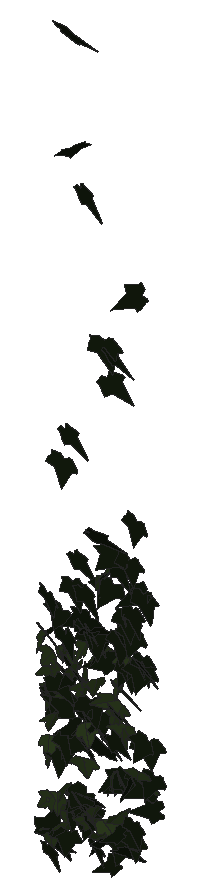
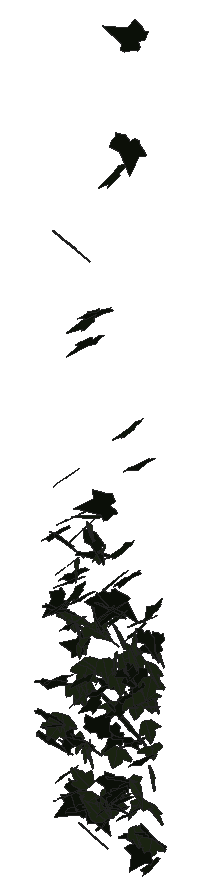
# SketchUp Ruby script. Lengths in inches.
U = 1.inch
M = Sketchup.active_model
def pt(a) = Geom::Point3d.new(a.map { |v| v * U })
def face(e, loops, mat)
  f = e.add_face(loops[0].map { |a| pt(a) })
  loops[1..].each { |l| e.add_face(l.map { |a| pt(a) }).erase! }
  f.material = f.back_material = mat if mat
  f
end
# faces: each face lists its corners as indices into pts; further lists are holes
def faces(e, pts, list, mat = nil) = list.each { |f| face(e, (f[0].is_a?(Array) ? f : [f]).map { |l| l.map { |i| pts[i] } }, mat) }
# xy, xz, yz: faces in a plane at the given z, y or x. An outline is a flat list of corners, or four numbers for a rectangle; further outlines are holes
def ring(l) = l.size == 4 ? [[l[0], l[1]], [l[2], l[1]], [l[2], l[3]], [l[0], l[3]]] : l.each_slice(2).to_a
def flat(e, list, mat, &to3) = list.each { |f| face(e, (f[0].is_a?(Array) ? f : [f]).map { |l| ring(l).map { |u, v| to3.(u, v) } }, mat) }
def xy(e, z, list, mat = nil) = flat(e, list, mat) { |x, y| [x, y, z] }
def xz(e, y, list, mat = nil) = flat(e, list, mat) { |x, z| [x, y, z] }
def yz(e, x, list, mat = nil) = flat(e, list, mat) { |y, z| [x, y, z] }
def lines(e, pts, list) = list.each { |a, b| e.add_line(pt(pts[a]), pt(pts[b])) }
# prism: a flat outline (further loops are holes) pulled along v
def prism(e, loops, v, mat = nil)
  f = face(e, loops, mat); d = Geom::Vector3d.new(v.map { |x| x * U })
  f.pushpull(f.normal.samedirection?(d) ? d.length : -d.length)
end
def box(e, o, s, mat = nil) = prism(e, [[o, [o[0] + s[0], o[1], o[2]], [o[0] + s[0], o[1] + s[1], o[2]], [o[0], o[1] + s[1], o[2]]]], [0, 0, s[2]], mat)
def at(x, y, z, deg = 0) = Geom::Transformation.translation(pt([x, y, z])) * Geom::Transformation.rotation(ORIGIN, Z_AXIS, deg.degrees)
def axes(o, x, y, z) = Geom::Transformation.new([*x, 0, *y, 0, *z, 0, *pt(o).to_a, 1])
def part(name) = M.definitions.add(name)
# library, detail: a bought-in or finely detailed component or shape, given as its bounding box
def library(name, o, s) = part(name).tap { |d| box(d.entities, o, s) }
def detail(e, o, s) = box(e.add_group.entities, o, s)
def put(e, d, t, mat = nil) = e.add_instance(d, t).tap { |i| i.material = mat if mat }
def group(e, t, mat = nil) = e.add_group.tap { |g| g.transformation = t; g.material = mat if mat }.entities
root = M.entities
M.materials.add("1026 AP 7946 SUNNY SIDE UP").color = [254, 231, 186]
M.materials.add("efeu1").color = [18, 25, 13]
M.materials.add("efeu2").color = [43, 57, 29]
c1 = part("ivyleaf_10")
p = [[0,0.5,-0.03],[-0.0625,2.02,-0.43],[-0.19,2.01,-0.46],[-0.54,1.05,-0.29],[-0.52,0.625,-0.18],[-0.83,0.76,-0.28],
  [-1.16,0.64,-0.33],[-1.15,0.33,-0.24],[-0.77,-0.39,0.02],[-0.3,-0.51,0.16],[0.04,-0.48,0.23],[-0.02,2.01,-0.4375],
  [-0.06,2.01,-0.43],[0.04,-0.49,0.23],[0.67,-0.49,0.14],[1.38,0.36,-0.2],[1.375,0.51,-0.24],[0.81,0.65,-0.19],
  [0.62,0.59,-0.15],[0.6,1.09,-0.28],[0.5,1.23,-0.31]]
faces(c1.entities,p,[[0,1,2,3,4,5,6,7,8,9,10],[11,12,0,13,14,15,16,17,18,19,20]],"efeu2")
c2 = part("ivyleaf_9")
p = [[1.54,2.16,1.25],[1.36,2.04,1.19],[-0.21,0.99,0.68],[-0.71,1.11,0.82],[-0.85,0.86,0.67],[-0.8,0.17,0.21],
  [-0.9,-0.01,0.1],[-0.67,-0.16,-0.02],[-0.08,-0.08,-0.05],[-0.03,-0.6,-0.4],[0.65,-0.88,-0.66],[0.83,-0.6,-0.49],
  [1.29,-0.42,-0.43],[1.8125,-0.07,-0.26],[1.21,0.44,0.15]]
faces(c2.entities,p,[[0,1,2,3,4,5,6,7,8,9,10,11,12,13,14]],"efeu1")
put(root,c1,axes([146.61,212.41,301.64],[0.32914,-0.30636,0.13113],[0.08129,-0.12062,-0.38215],[0.51634,0.21427,-0.02343]),"1026 AP 7946 SUNNY SIDE UP")
put(root,c1,axes([146.92,212.51,295.66],[0.25762,-0.30864,-0.15791],[-0.06539,0.14883,-0.35776],[0.53668,0.16629,0.03221]),"1026 AP 7946 SUNNY SIDE UP")
put(root,c1,axes([146.98,212.42,300.85],[0.4916,-0.19284,-0.1642],[-0.176,0.11838,-0.37564],[0.35059,0.32983,0.04166]),"1026 AP 7946 SUNNY SIDE UP")
put(root,c1,axes([147.09,212.25,293.68],[0.41654,-0.20792,-0.16591],[-0.21468,0.08468,-0.34604],[0.35211,0.29759,-0.01472]),"1026 AP 7946 SUNNY SIDE UP")
put(root,c2,axes([146.62,212.33,302.03],[0.47433,-0.25687,0.06374],[0.04272,-0.06546,-0.40723],[0.41379,0.3012,-0.03102]),"1026 AP 7946 SUNNY SIDE UP")
put(root,c1,axes([147,212.45,300.1],[-0.32461,-0.31438,-0.10633],[0.11674,0.0724,-0.3864],[0.50614,-0.21833,0.02092]),"1026 AP 7946 SUNNY SIDE UP")
put(root,c1,axes([147.26,211.93,298.96],[0.12832,-0.10009,-0.39365],[-0.2696,0.34189,-0.12817],[0.55857,0.18801,0.02857]),"1026 AP 7946 SUNNY SIDE UP")
put(root,c2,axes([146.75,212.5625,303.73],[0.11591,-0.34584,0.20587],[0.04419,-0.20022,-0.36523],[0.62805,0.07791,-0.01229]),"1026 AP 7946 SUNNY SIDE UP")
put(root,c2,axes([146.77,212.61,290.94],[0.19947,-0.32596,0.04859],[0.01514,-0.04883,-0.36051],[0.51808,0.12693,-0.00817]),"1026 AP 7946 SUNNY SIDE UP")
put(root,c1,axes([147.08,212.35,291.9],[-0.52664,-0.12026,-0.02486],[0.05589,-0.03006,-0.36444],[0.18437,-0.3344,0.03947]),"1026 AP 7946 SUNNY SIDE UP")
put(root,c2,axes([147.35,212.35,302.3],[-0.17953,0.38066,0.00946],[-0.02951,0.00169,-0.40901],[-0.59793,-0.11438,0.01735]),"1026 AP 7946 SUNNY SIDE UP")
put(root,c2,axes([147.09,212.21,292.05],[-0.52102,0.26292,0.10411],[0.15602,-0.03462,0.43418],[0.41361,0.34425,-0.03264]),"1026 AP 7946 SUNNY SIDE UP")
put(root,c1,axes([147.22,212.4,297.79],[-0.15938,-0.36666,0.03818],[-0.00244,-0.04017,-0.39202],[0.57981,-0.10096,0.00884]),"1026 AP 7946 SUNNY SIDE UP")
put(root,c1,axes([147.11,212.21,296.65],[0.29945,0.31816,-0.08585],[-0.04014,-0.0838,-0.38189],[-0.51632,0.19104,-0.0201]),"1026 AP 7946 SUNNY SIDE UP")
put(root,c1,axes([147.375,212.48,299.29],[-0.39187,-0.26307,0.1613],[-0.11352,-0.14765,-0.37128],[0.46903,-0.25552,0.0449]),"1026 AP 7946 SUNNY SIDE UP")
put(root,c2,axes([147.33,212.59,299],[-0.22007,-0.34448,0.1264],[0.00308,-0.13414,-0.38042],[0.57603,-0.13089,0.05033]),"1026 AP 7946 SUNNY SIDE UP")
put(root,c2,axes([147.54,212.63,298.7],[-0.43764,-0.24619,0.11937],[0.02108,-0.17971,-0.35695],[0.42826,-0.24273,0.13955]),"1026 AP 7946 SUNNY SIDE UP")
put(root,c2,axes([147.41,212.73,303.05],[-0.24174,-0.32129,0.18276],[0.02428,-0.19971,-0.35635],[0.57798,-0.12599,0.09141]),"1026 AP 7946 SUNNY SIDE UP")
put(root,c2,axes([147.39,212.47,291.4],[0.53282,0.05427,-0.09357],[-0.1364,-0.03377,-0.35319],[-0.09597,0.34927,-0.0175]),"1026 AP 7946 SUNNY SIDE UP")
put(root,c2,axes([147.47,212.5,296.03],[-0.10423,-0.36939,0.04016],[0.00163,-0.04192,-0.38677],[0.5844,-0.06577,0.00824]),"1026 AP 7946 SUNNY SIDE UP")
put(root,c2,axes([147.39,212.37,299.73],[0.10569,-0.3293,-0.2036],[0.05786,0.20338,-0.33824],[0.59959,0.03842,0.06853]),"1026 AP 7946 SUNNY SIDE UP")
put(root,c1,axes([147.75,212.58,292.375],[-0.17222,-0.33626,0.0407],[-0.00934,-0.04162,-0.3645],[0.53265,-0.10945,0.00677]),"1026 AP 7946 SUNNY SIDE UP")
put(root,c1,axes([147.51,212.29,293.87],[0.52255,-0.10033,0.14238],[0.19128,-0.07492,-0.35635],[0.18952,0.35226,-0.03292]),"1026 AP 7946 SUNNY SIDE UP")
put(root,c1,axes([147.81,212.54,298.81],[-0.41678,-0.2879,0.03723],[0.05352,-0.08159,-0.39513],[0.45343,-0.255,0.08085]),"1026 AP 7946 SUNNY SIDE UP")
put(root,c1,axes([147.82,212.65,301.33],[0.03837,-0.39672,0.015],[-0.00117,-0.01689,-0.40957],[0.62437,0.02435,-0.00169]),"1026 AP 7946 SUNNY SIDE UP")
put(root,c2,axes([147.34,212.68,300.18],[0.47768,-0.27922,0.15131],[0.13332,-0.12642,-0.4244],[0.47904,0.3136,-0.03277]),"1026 AP 7946 SUNNY SIDE UP")
put(root,c2,axes([147.69,212.51,310.8],[-0.14697,-0.41525,0.06499],[0.00015,-0.06706,-0.43862],[0.661,-0.09231,0.01455]),"1026 AP 7946 SUNNY SIDE UP")
put(root,c1,axes([147.64,212.79,301.86],[0.10847,-0.09427,0.38721],[0.35279,-0.30222,-0.12211],[0.49779,0.23473,0.00216]),"1026 AP 7946 SUNNY SIDE UP")
put(root,c2,axes([148.32,212.32,298.52],[-0.14329,0.07953,0.3839],[-0.57865,-0.11606,-0.06795],[0.15269,-0.3652,0.10274]),"1026 AP 7946 SUNNY SIDE UP")
put(root,c1,axes([148,212.14,293.4],[-0.04686,0.1928,0.33057],[-0.14966,0.30629,-0.19758],[-0.56776,-0.09665,0.0248]),"1026 AP 7946 SUNNY SIDE UP")
put(root,c2,axes([147.91,212.54,292.1],[-0.28081,-0.30375,-0.06359],[0.07712,0.04063,-0.36209],[0.48069,-0.18396,0.02094]),"1026 AP 7946 SUNNY SIDE UP")
put(root,c1,axes([148.07,212.29,294.57],[0.08603,-0.34987,0.13121],[0.0066,-0.13015,-0.36525],[0.58649,0.05278,-0.01514]),"1026 AP 7946 SUNNY SIDE UP")
put(root,c2,axes([148.24,212.51,300.19],[-0.50665,0.17142,-0.14232],[0.16477,-0.09789,-0.37486],[-0.30555,-0.33704,0.03384]),"1026 AP 7946 SUNNY SIDE UP")
put(root,c2,axes([147.92,212.55,296.76],[-0.13044,-0.36822,0.06212],[0.01498,-0.06598,-0.38848],[0.58706,-0.08013,0.02372]),"1026 AP 7946 SUNNY SIDE UP")
put(root,c2,axes([148.39,212.5,297.63],[-0.45366,0.2521,0.00125],[-0.02633,-0.0195,-0.39393],[-0.39552,-0.28785,0.02479]),"1026 AP 7946 SUNNY SIDE UP")
put(root,c2,axes([148.24,212.38,326.78],[0.15242,0.45673,-0.01275],[-0.00964,-0.01401,-0.48107],[-0.71849,0.09708,0.00375]),"1026 AP 7946 SUNNY SIDE UP")
put(root,c2,axes([147.86,212.36,302.26],[0.13053,-0.39204,0.05276],[0.0004,-0.05455,-0.413],[0.62215,0.08229,-0.0108]),"1026 AP 7946 SUNNY SIDE UP")
put(root,c1,axes([147.73,212.55,301.24],[0.44272,-0.07151,0.284],[0.44777,0.04933,-0.28573],[0.02446,0.39123,0.09034]),"1026 AP 7946 SUNNY SIDE UP")
put(root,c2,axes([148,212.82,293.24],[-0.08719,-0.35007,0.08808],[-0.0018,-0.08834,-0.36543],[0.56737,-0.05408,0.01238]),"1026 AP 7946 SUNNY SIDE UP")
put(root,c2,axes([147.81,212.62,300.57],[0.50294,-0.23192,0.02177],[0.02629,-0.01518,-0.4071],[0.36543,0.32028,-0.00068]),"1026 AP 7946 SUNNY SIDE UP")
put(root,c2,axes([147.59,212.7,332.3125],[0.36792,-0.25152,0.34328],[0.44603,-0.18669,-0.34997],[0.4841,0.36316,0.06155]),"1026 AP 7946 SUNNY SIDE UP")
put(root,c2,axes([147.9,212.43,300.95],[0.36799,-0.31633,0.05833],[0.01737,-0.0643,-0.40464],[0.50551,0.23249,-0.02856]),"1026 AP 7946 SUNNY SIDE UP")
put(root,c2,axes([148.33,212.74,296.92],[-0.53188,-0.17299,-0.03841],[0.09314,-0.03708,-0.38675],[0.26187,-0.33818,0.05954]),"1026 AP 7946 SUNNY SIDE UP")
put(root,c2,axes([148.03,212.32,312.5],[0.34935,-0.36087,-0.12526],[-0.038,0.12477,-0.43358],[0.59655,0.21928,0.04573]),"1026 AP 7946 SUNNY SIDE UP")
put(root,c1,axes([148.47,212.47,300.75],[-0.04407,-0.40064,0.00917],[0.00009,-0.01121,-0.41381],[0.63021,-0.02802,0.0007]),"1026 AP 7946 SUNNY SIDE UP")
put(root,c2,axes([148.37,212.85,293.9],[-0.17268,-0.30766,0.16781],[0.02477,-0.1768,-0.33057],[0.54813,-0.08894,0.06781]),"1026 AP 7946 SUNNY SIDE UP")
put(root,c2,axes([148.3,212.41,304.87],[0.03203,-0.41067,-0.06075],[-0.02503,0.05589,-0.42305],[0.65137,0.02234,-0.01327]),"1026 AP 7946 SUNNY SIDE UP")
put(root,c2,axes([148.39,212.81,293.42],[-0.18603,-0.33933,0.01923],[0.1223,-0.04825,-0.35892],[0.52037,-0.10997,0.09123]),"1026 AP 7946 SUNNY SIDE UP")
put(root,c2,axes([148.32,212.63,298.49],[0.43961,-0.25969,-0.03515],[-0.05066,0.01326,-0.39282],[0.40842,0.28117,-0.01089]),"1026 AP 7946 SUNNY SIDE UP")
put(root,c2,axes([148.66,212.55,294.25],[-0.26719,-0.28485,0.16004],[-0.08023,-0.15156,-0.34113],[0.50507,-0.17477,0.03047]),"1026 AP 7946 SUNNY SIDE UP")
put(root,c1,axes([148.77,212.62,299.76],[-0.1948,-0.36797,0.06551],[0.0076,-0.07076,-0.39945],[0.5877,-0.12105,0.02688]),"1026 AP 7946 SUNNY SIDE UP")
put(root,c2,axes([148.46,212.4375,306.26],[0.3315,-0.34362,-0.09324],[0.00493,0.10481,-0.41065],[0.55794,0.20323,0.05903]),"1026 AP 7946 SUNNY SIDE UP")
put(root,c2,axes([148.96,212.4,294.52],[-0.51811,-0.16493,0.0338],[-0.01048,-0.06133,-0.37621],[0.2645,-0.3255,0.0513]),"1026 AP 7946 SUNNY SIDE UP")
put(root,c1,axes([148.84,212.56,295.99],[-0.57454,-0.10058,-0.02897],[0.06642,-0.05094,-0.38577],[0.14993,-0.36287,0.05986]),"1026 AP 7946 SUNNY SIDE UP")
put(root,c2,axes([148.56,212.4,294.16],[0.37487,-0.27835,0.03797],[0.00469,-0.0479,-0.37668],[0.44181,0.23669,-0.02822]),"1026 AP 7946 SUNNY SIDE UP")
put(root,c2,axes([148.6,212.59,302.89],[0.21562,-0.38131,-0.00722],[-0.00757,0.00342,-0.41742],[0.59958,0.13717,-0.00267]),"1026 AP 7946 SUNNY SIDE UP")
put(root,c1,axes([148.92,212.38,301.95],[0.40489,-0.30775,0.00224],[-0.02733,-0.01965,-0.41264],[0.48318,0.25678,-0.02522]),"1026 AP 7946 SUNNY SIDE UP")
put(root,c2,axes([148.75,212.52,296.93],[0.52038,-0.12946,-0.14012],[-0.21921,0.01302,-0.36412],[0.19654,0.35729,-0.03513]),"1026 AP 7946 SUNNY SIDE UP")
put(root,c2,axes([149.33,212.23,303.54],[0.13033,0.03526,-0.43759],[-0.55346,-0.23873,-0.09253],[-0.37851,0.36121,-0.01538]),"1026 AP 7946 SUNNY SIDE UP")
put(root,c1,axes([148.83,212.59,300.68],[0.23521,-0.36264,-0.00024],[0.17692,0.04453,-0.38416],[0.54208,0.14281,0.12548]),"1026 AP 7946 SUNNY SIDE UP")
put(root,c2,axes([149.32,212.69,293.31],[-0.14717,0.03442,0.36684],[-0.53842,-0.11454,-0.08203],[0.16185,-0.34972,0.06069]),"1026 AP 7946 SUNNY SIDE UP")
put(root,c2,axes([149.03,212.35,294.34],[0.479,0.15612,-0.14267],[-0.23083,-0.01601,-0.34913],[-0.23453,0.33461,0.05225]),"1026 AP 7946 SUNNY SIDE UP")
put(root,c2,axes([148.8,212.49,304.65],[0.23233,-0.38036,-0.07542],[-0.03124,0.06849,-0.41993],[0.60763,0.14896,0.00725]),"1026 AP 7946 SUNNY SIDE UP")
put(root,c1,axes([149.26,212.39,293.26],[-0.4991,-0.17481,0.01506],[0.00091,-0.0333,-0.37227],[0.27596,-0.31605,0.02846]),"1026 AP 7946 SUNNY SIDE UP")
put(root,c2,axes([149.18,212.64,293.28],[-0.46558,-0.14389,-0.15467],[0.25892,-0.00493,-0.33152],[0.1982,-0.33158,0.06974]),"1026 AP 7946 SUNNY SIDE UP")
put(root,c2,axes([149.49,212.42,298.32],[-0.51219,0.20755,-0.08453],[0.07482,-0.07936,-0.39618],[-0.34357,-0.3267,0.03974]),"1026 AP 7946 SUNNY SIDE UP")
put(root,c2,axes([149.05,212.625,303.02],[-0.04076,-0.39616,0.08129],[0.00767,-0.08163,-0.40934],[0.63581,-0.02441,0.01015]),"1026 AP 7946 SUNNY SIDE UP")
put(root,c2,axes([148.94,212.28,324.93],[0.40234,-0.38882,-0.0875],[-0.0795,0.06575,-0.47909],[0.62,0.26075,-0.00465]),"1026 AP 7946 SUNNY SIDE UP")
put(root,c1,axes([149.33,212.6,293.71],[-0.11965,-0.36597,0.02168],[0.00682,-0.02451,-0.38511],[0.57656,-0.07566,0.00905]),"1026 AP 7946 SUNNY SIDE UP")
put(root,c1,axes([149.42,212.44,293.22],[-0.2457,-0.31765,0.0729],[-0.03715,-0.06923,-0.36498],[0.511,-0.15777,0.00852]),"1026 AP 7946 SUNNY SIDE UP")
put(root,c2,axes([149.17,212.33,293.42],[0.39499,-0.17005,-0.21771],[-0.21978,0.16419,-0.30771],[0.36415,0.28354,0.05043]),"1026 AP 7946 SUNNY SIDE UP")
put(root,c1,axes([149.45,212.625,300.21],[-0.20427,-0.37273,0.0124],[0.01409,-0.0181,-0.40648],[0.58634,-0.12942,0.01409]),"1026 AP 7946 SUNNY SIDE UP")
put(root,c1,axes([149.27,212.11,298.02],[0.29444,0.34271,0.0016],[0.02465,-0.00901,-0.40194],[-0.53831,0.18704,-0.01753]),"1026 AP 7946 SUNNY SIDE UP")
put(root,c2,axes([149.27,212.45,299.2],[-0.2967,-0.2459,-0.24452],[0.43027,0.05145,-0.28036],[0.31942,-0.29771,0.15054]),"1026 AP 7946 SUNNY SIDE UP")
put(root,c2,axes([149.3,212.54,302.84],[0.24806,-0.36312,0.0444],[0.00516,-0.04777,-0.40781],[0.57535,0.15699,-0.01549]),"1026 AP 7946 SUNNY SIDE UP")
put(root,c2,axes([149.59,212.18,303.01],[0.46996,0.26697,-0.05666],[-0.03208,-0.06173,-0.41189],[-0.42788,0.29785,-0.03136]),"1026 AP 7946 SUNNY SIDE UP")
put(root,c2,axes([149.85,212.65,296.72],[0.37146,-0.13926,0.27463],[-0.33027,0.16764,0.28211],[-0.34004,-0.31495,0.026]),"1026 AP 7946 SUNNY SIDE UP")
put(root,c2,axes([149.56,212.29,302.85],[-0.35701,-0.22772,-0.23964],[0.35738,0.09002,-0.32059],[0.36441,-0.31138,0.07962]),"1026 AP 7946 SUNNY SIDE UP")
put(root,c2,axes([149.57,212.42,292.12],[0.13916,-0.30811,0.17035],[0.05098,-0.16441,-0.33096],[0.54878,0.0934,-0.01245]),"1026 AP 7946 SUNNY SIDE UP")
put(root,c1,axes([150.09,212.7,301.84],[0.34654,0.15271,-0.30202],[-0.43093,-0.11443,-0.27351],[-0.29277,0.34919,0.0451]),"1026 AP 7946 SUNNY SIDE UP")
put(root,c2,axes([150.05,212.42,292.49],[-0.06338,0.29391,-0.21349],[0.02277,-0.20871,-0.30661],[-0.56653,-0.04127,0.01156]),"1026 AP 7946 SUNNY SIDE UP")
put(root,c2,axes([149.99,212.55,302.39],[-0.41308,0.15151,-0.26388],[0.32237,-0.15709,-0.31222],[-0.34079,-0.33225,0.0245]),"1026 AP 7946 SUNNY SIDE UP")
put(root,c1,axes([149.875,212.29,305.6],[-0.0259,0.39027,-0.09004],[0.00089,-0.08967,-0.40292],[-0.62963,-0.01618,0.00314]),"1026 AP 7946 SUNNY SIDE UP")
put(root,c1,axes([149.71,212.55,292.43],[-0.24183,-0.25859,0.20974],[0.27556,0.12772,0.30207],[-0.43974,0.22224,0.07394]),"1026 AP 7946 SUNNY SIDE UP")
put(root,c2,axes([149.83,212.59,298.72],[-0.09757,-0.37907,0.04153],[-0.00531,-0.04248,-0.39594],[0.59975,-0.06204,0.00325]),"1026 AP 7946 SUNNY SIDE UP")
put(root,c2,axes([150.49,212.32,301.69],[-0.54014,0.17385,0.08616],[-0.15,-0.00689,-0.39355],[-0.2629,-0.35325,0.04751]),"1026 AP 7946 SUNNY SIDE UP")
put(root,c2,axes([149.61,212.125,307.91],[0.59312,-0.05978,0.19009],[0.28455,-0.0388,-0.39356],[0.11116,0.41828,-0.00682]),"1026 AP 7946 SUNNY SIDE UP")
put(root,c2,axes([150.39,212.29,306.18],[-0.16734,0.38746,0.02961],[-0.01587,0.02475,-0.41379],[-0.61047,-0.10685,0.00264]),"1026 AP 7946 SUNNY SIDE UP")
put(root,c1,axes([150.55,212.36,299.75],[0.34406,0.07319,-0.33224],[-0.51577,-0.00485,-0.23014],[-0.07098,0.39004,0.06185]),"1026 AP 7946 SUNNY SIDE UP")
put(root,c2,axes([150.07,212.42,317.61],[-0.07877,-0.44127,-0.0831],[0.08915,0.07177,-0.45447],[0.69899,-0.05888,0.0486]),"1026 AP 7946 SUNNY SIDE UP")
put(root,c1,axes([150.05,212.52,293.25],[0.38136,0.21656,0.18729],[0.2405,0.09904,-0.33343],[-0.37246,0.28569,-0.02354]),"1026 AP 7946 SUNNY SIDE UP")
put(root,c2,axes([150.4,212.55,305.43],[-0.47104,-0.27468,0.01991],[0.05335,-0.06741,-0.41238],[0.42985,-0.29263,0.073]),"1026 AP 7946 SUNNY SIDE UP")
put(root,c1,axes([150.41,212.61,295.48],[0.25756,-0.33155,-0.03963],[-0.03577,0.02956,-0.38072],[0.52327,0.16521,-0.00652]),"1026 AP 7946 SUNNY SIDE UP")
put(root,c2,axes([150.72,212.49,291.51],[-0.49178,0.18503,0.02243],[-0.05237,-0.01574,-0.37314],[-0.28803,-0.31305,0.02954]),"1026 AP 7946 SUNNY SIDE UP")
put(root,c1,axes([150.43,212.43,306.57],[0.30764,-0.35283,-0.01322],[-0.02983,0.00186,-0.4153],[0.55425,0.19594,-0.01502]),"1026 AP 7946 SUNNY SIDE UP")
put(root,c2,axes([150.11,212.25,298],[0.47177,-0.26512,-0.05323],[-0.08394,0.01522,-0.41165],[0.41589,0.30381,-0.0227]),"1026 AP 7946 SUNNY SIDE UP")
put(root,c1,axes([150.52,212.45,295.67],[-0.13133,0.36155,0.09268],[-0.1261,0.07049,-0.37673],[-0.57131,-0.09867,0.06185]),"1026 AP 7946 SUNNY SIDE UP")
put(root,c1,axes([150.53,212.55,299.04],[0.46849,-0.25233,-0.00686],[0.03638,0.03536,-0.39969],[0.39518,0.29588,0.04493]),"1026 AP 7946 SUNNY SIDE UP")
put(root,c1,axes([150.61,212.54,299.41],[-0.59776,0.03754,-0.05159],[0.06877,-0.06292,-0.38938],[-0.07077,-0.37827,0.05735]),"1026 AP 7946 SUNNY SIDE UP")
put(root,c2,axes([150.29,212.48,317.24],[0.46799,-0.31862,-0.11776],[-0.06027,0.11711,-0.44549],[0.52788,0.29584,0.05353]),"1026 AP 7946 SUNNY SIDE UP")
put(root,c2,axes([150.73,212.47,307.1],[-0.52094,-0.21865,0.14213],[0.01076,-0.23321,-0.36195],[0.40743,-0.2734,0.19129]),"1026 AP 7946 SUNNY SIDE UP")
put(root,c2,axes([150.4375,212.42,299.42],[0.50278,-0.15764,-0.16783],[-0.18584,0.12266,-0.36253],[0.30299,0.33682,0.05614]),"1026 AP 7946 SUNNY SIDE UP")
put(root,c2,axes([150.97,212.5625,295.91],[-0.58784,0.02492,-0.00673],[0.00662,-0.03672,-0.38438],[-0.04002,-0.3721,0.03528]),"1026 AP 7946 SUNNY SIDE UP")
put(root,c2,axes([150.49,212.22,316],[0.23829,-0.30873,-0.30132],[-0.03353,0.3028,-0.34093],[0.66598,0.12571,0.09065]),"1026 AP 7946 SUNNY SIDE UP")
put(root,c1,axes([150.66,212.43,293.71],[-0.1129,-0.34529,0.16981],[0.14285,0.14955,0.36009],[-0.5858,0.10301,0.05508]),"1026 AP 7946 SUNNY SIDE UP")
put(root,c1,axes([150.79,212.62,300.64],[-0.01134,-0.28612,0.27176],[0.18223,-0.25506,-0.2815],[0.58598,0.07378,0.0928]),"1026 AP 7946 SUNNY SIDE UP")
put(root,c2,axes([150.65,212.48,306.57],[0.24661,-0.3522,-0.12533],[-0.08695,0.10634,-0.39649],[0.57838,0.16615,-0.00617]),"1026 AP 7946 SUNNY SIDE UP")
put(root,c1,axes([150.88,212.49,295.89],[-0.34715,0.3023,0.01428],[-0.02444,0.00368,-0.38547],[-0.47509,-0.22108,0.0094]),"1026 AP 7946 SUNNY SIDE UP")
put(root,c2,axes([151.2,212.24,293.32],[-0.43844,0.23662,-0.01934],[-0.01497,-0.04215,-0.37493],[-0.37311,-0.27636,0.03778]),"1026 AP 7946 SUNNY SIDE UP")
put(root,c1,axes([150.84,212.57,298.27],[-0.47679,0.21663,-0.11085],[0.09783,-0.09891,-0.38198],[-0.36843,-0.30661,0.04203]),"1026 AP 7946 SUNNY SIDE UP")
put(root,c1,axes([151.07,212.58,298.45],[-0.40187,-0.26046,0.13685],[-0.08092,-0.13557,-0.37248],[0.45364,-0.25492,0.05479]),"1026 AP 7946 SUNNY SIDE UP")
put(root,c2,axes([150.9,212.73,292.53],[-0.25359,-0.32531,0.03935],[-0.0246,-0.03694,-0.37426],[0.51478,-0.16202,0.0015]),"1026 AP 7946 SUNNY SIDE UP")
put(root,c2,axes([150.8125,212.07,298.14],[0.28157,-0.25515,-0.24056],[-0.14472,0.21664,-0.31728],[0.52265,0.19745,0.04175]),"1026 AP 7946 SUNNY SIDE UP")
put(root,c2,axes([151.4,212.74,295.71],[-0.533,-0.08753,0.13961],[-0.19157,-0.06957,-0.35933],[0.16729,-0.35856,0.03334]),"1026 AP 7946 SUNNY SIDE UP")
put(root,c2,axes([150.96,212.5,302.91],[-0.09934,-0.38756,0.09886],[-0.00272,-0.09912,-0.40486],[0.62863,-0.06167,0.01387]),"1026 AP 7946 SUNNY SIDE UP")
put(root,c2,axes([150.95,212.4375,303.33],[0.42625,-0.23741,-0.1793],[-0.16711,0.13976,-0.36897],[0.43031,0.28944,0.03432]),"1026 AP 7946 SUNNY SIDE UP")
put(root,c1,axes([151.27,212.26,304.44],[-0.26597,0.35202,0.09955],[-0.16527,0.05279,-0.39554],[-0.54882,-0.18649,0.07087]),"1026 AP 7946 SUNNY SIDE UP")
put(root,c1,axes([151.3125,212.29,301.34],[0.27624,-0.35903,-0.02021],[-0.01964,0.01345,-0.41166],[0.56487,0.17604,-0.00443]),"1026 AP 7946 SUNNY SIDE UP")
put(root,c2,axes([150.87,212.4375,300.5],[0.33876,-0.27893,0.17015],[0.19158,-0.11613,-0.36299],[0.47371,0.24643,0.02513]),"1026 AP 7946 SUNNY SIDE UP")
put(root,c2,axes([151.3,212.64,301.74],[-0.53412,-0.11956,-0.17784],[0.31224,-0.07976,-0.34746],[0.10464,-0.37228,0.12906]),"1026 AP 7946 SUNNY SIDE UP")
put(root,c2,axes([151.49,211.93,292.9],[0.06015,0.34119,0.13412],[0.00594,0.12857,-0.35279],[-0.5731,0.03714,0.01042]),"1026 AP 7946 SUNNY SIDE UP")
put(root,c2,axes([151.11,212.26,292.41],[0.47468,0.16635,0.12458],[0.18156,0.03863,-0.35423],[-0.26656,0.32255,-0.01942]),"1026 AP 7946 SUNNY SIDE UP")
put(root,c1,axes([151.27,212.54,301.875],[0.606,0.09528,0.01247],[0.02574,-0.01809,-0.4085],[-0.14871,0.38515,-0.01987]),"1026 AP 7946 SUNNY SIDE UP")
put(root,c2,axes([151.23,212.61,304.15],[-0.0834,-0.40493,-0.02187],[-0.0011,0.01919,-0.4206],[0.63741,-0.05295,-0.00358]),"1026 AP 7946 SUNNY SIDE UP")
put(root,c2,axes([151.24,212.63,301.64],[-0.019,-0.39863,0.01696],[-0.00097,-0.01872,-0.41097],[0.6275,-0.0121,-0.00012]),"1026 AP 7946 SUNNY SIDE UP")
put(root,c2,axes([151.39,212.78,295.85],[-0.14482,0.03549,-0.37324],[0.3533,-0.28875,-0.08962],[-0.45077,-0.23772,0.04967]),"1026 AP 7946 SUNNY SIDE UP")
put(root,c2,axes([151.3,212.6875,306.93],[-0.06127,-0.40807,0.06413],[0.05404,-0.06783,-0.42067],[0.64738,-0.03296,0.04118]),"1026 AP 7946 SUNNY SIDE UP")
put(root,c2,axes([151.45,212.78,292.95],[-0.08576,-0.35878,0.04842],[0.06091,-0.05509,-0.37115],[0.56613,-0.04842,0.04727]),"1026 AP 7946 SUNNY SIDE UP")
put(root,c2,axes([151.47,212.65,304.47],[0.07482,-0.40265,0.03797],[-0.0039,-0.03971,-0.41786],[0.6361,0.04712,-0.00703]),"1026 AP 7946 SUNNY SIDE UP")
put(root,c2,axes([151.55,212.81,308.88],[-0.06942,-0.37551,0.175],[-0.02115,-0.17159,-0.39047],[0.64911,-0.04575,0.006]),"1026 AP 7946 SUNNY SIDE UP")
put(root,c2,axes([152.12,212.37,320.6875],[-0.68071,0.15169,-0.02252],[0.0076,-0.05451,-0.47009],[-0.24106,-0.43007,0.04877]),"1026 AP 7946 SUNNY SIDE UP")
put(root,c2,axes([151.67,212.5,303.48],[-0.21074,-0.36802,0.12149],[0.01517,-0.13015,-0.40078],[0.60848,-0.12421,0.05207]),"1026 AP 7946 SUNNY SIDE UP")
put(root,c2,axes([152.17,212.51,305.63],[-0.62786,0.08591,-0.00502],[-0.00406,-0.03738,-0.41925],[-0.13528,-0.39758,0.03588]),"1026 AP 7946 SUNNY SIDE UP")
put(root,c2,axes([151.63,212.52,293.84],[0.05964,-0.36857,0.07334],[0.01885,-0.07243,-0.3821],[0.59059,0.03953,0.00479]),"1026 AP 7946 SUNNY SIDE UP")
put(root,c1,axes([152,212.44,296.5],[-0.58789,-0.01278,0.0538],[-0.07916,-0.04713,-0.38287],[0.03001,-0.37456,0.04411]),"1026 AP 7946 SUNNY SIDE UP")
put(root,c2,axes([152,212.73,302.18],[0.02148,-0.39737,0.01184],[-0.00812,-0.01394,-0.40965],[0.62515,0.01347,-0.00572]),"1026 AP 7946 SUNNY SIDE UP")
put(root,c2,axes([152.29,212.42,301.95],[-0.49348,-0.2162,-0.12247],[0.21115,0.00937,-0.38673],[0.32435,-0.33504,0.06543]),"1026 AP 7946 SUNNY SIDE UP")
put(root,c2,axes([152.56,212.51,295.92],[-0.47102,-0.12601,0.18348],[-0.17122,-0.17709,-0.31751],[0.29834,-0.30058,0.10746]),"1026 AP 7946 SUNNY SIDE UP")
put(root,c1,axes([152.29,212.49,295.95],[-0.54694,0.04416,-0.11808],[0.1664,-0.06844,-0.35765],[-0.09876,-0.35987,0.05131]),"1026 AP 7946 SUNNY SIDE UP")
put(root,c2,axes([152.43,212.45,298.28],[-0.29025,-0.3157,0.13358],[-0.0626,-0.12853,-0.37634],[0.53407,-0.18664,0.02848]),"1026 AP 7946 SUNNY SIDE UP")
put(root,c2,axes([152.18,212.16,302.27],[0.59001,-0.15193,-0.08428],[-0.13493,0.00321,-0.41598],[0.23466,0.38385,-0.02728]),"1026 AP 7946 SUNNY SIDE UP")
put(root,c2,axes([152.37,212.33,305.6875],[0.00854,-0.4139,-0.03092],[0.01044,0.02775,-0.42621],[0.65218,0.00498,0.00723]),"1026 AP 7946 SUNNY SIDE UP")
put(root,c2,axes([152.47,212.53,298.24],[-0.2766,-0.32619,-0.13084],[0.21615,0.0642,-0.37105],[0.50505,-0.20612,0.08714]),"1026 AP 7946 SUNNY SIDE UP")
put(root,c2,axes([152.69,212.6,296.52],[-0.49929,-0.12662,-0.1538],[0.24339,0.00952,-0.34912],[0.18701,-0.35044,0.04376]),"1026 AP 7946 SUNNY SIDE UP")
put(root,c2,axes([153.16,212.31,295.11],[-0.49609,0.11444,0.16123],[-0.24342,0.0292,-0.34477],[-0.18216,-0.35068,0.02163]),"1026 AP 7946 SUNNY SIDE UP")
